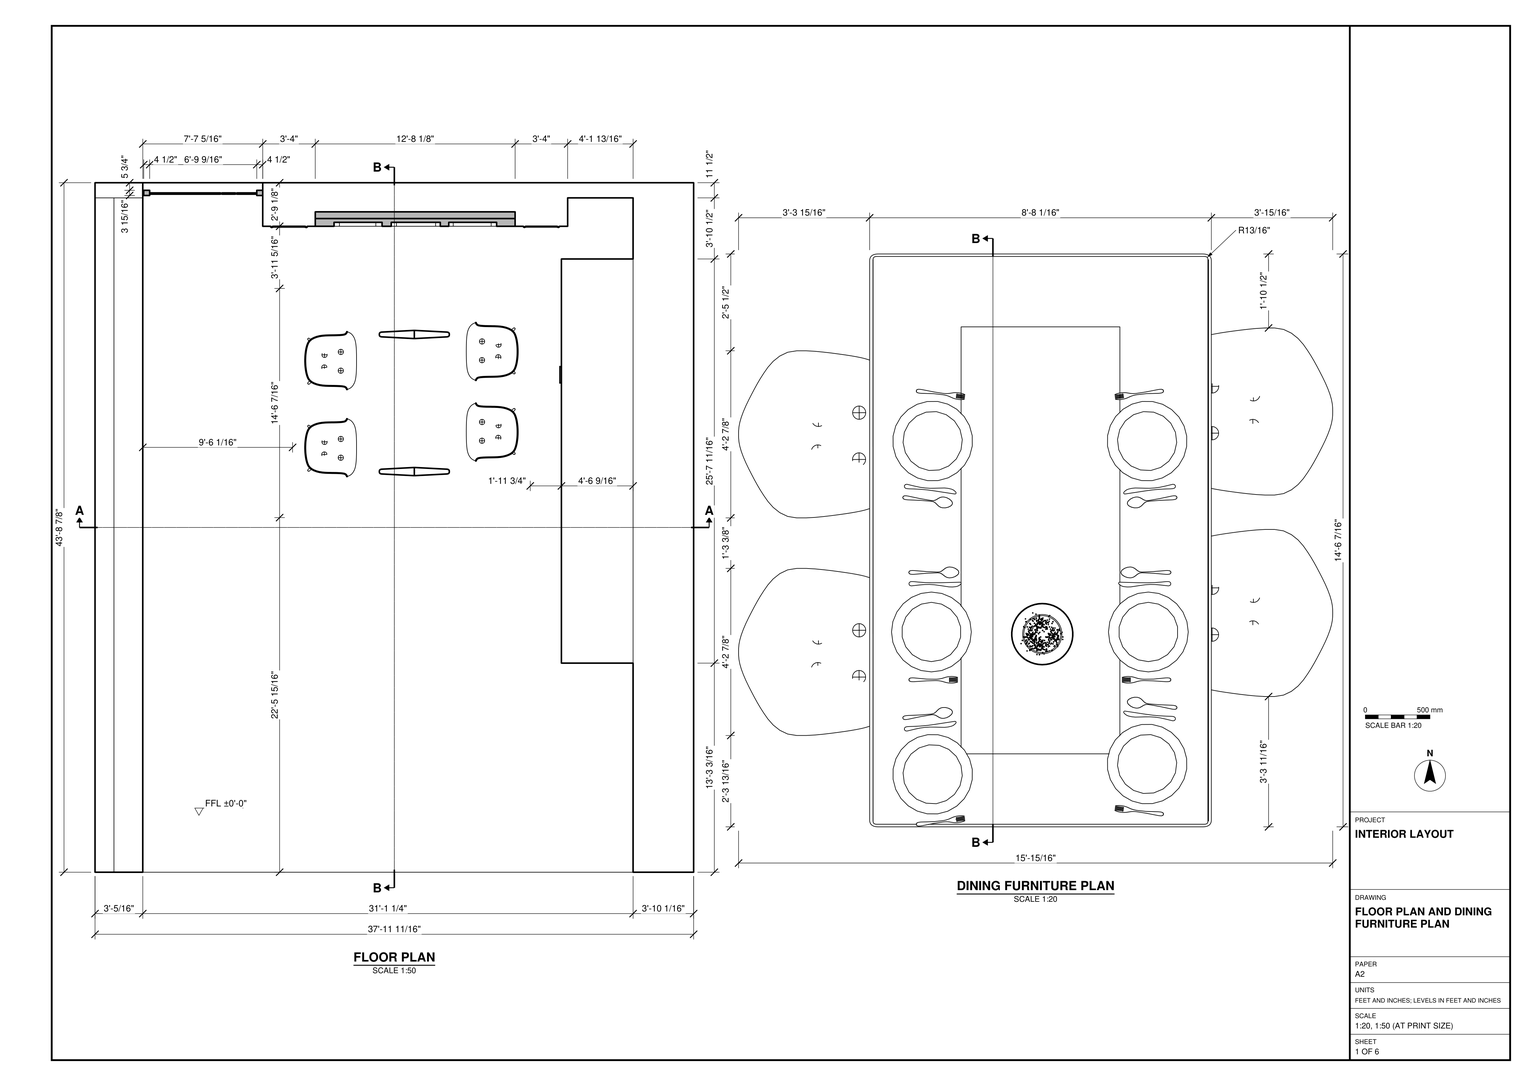
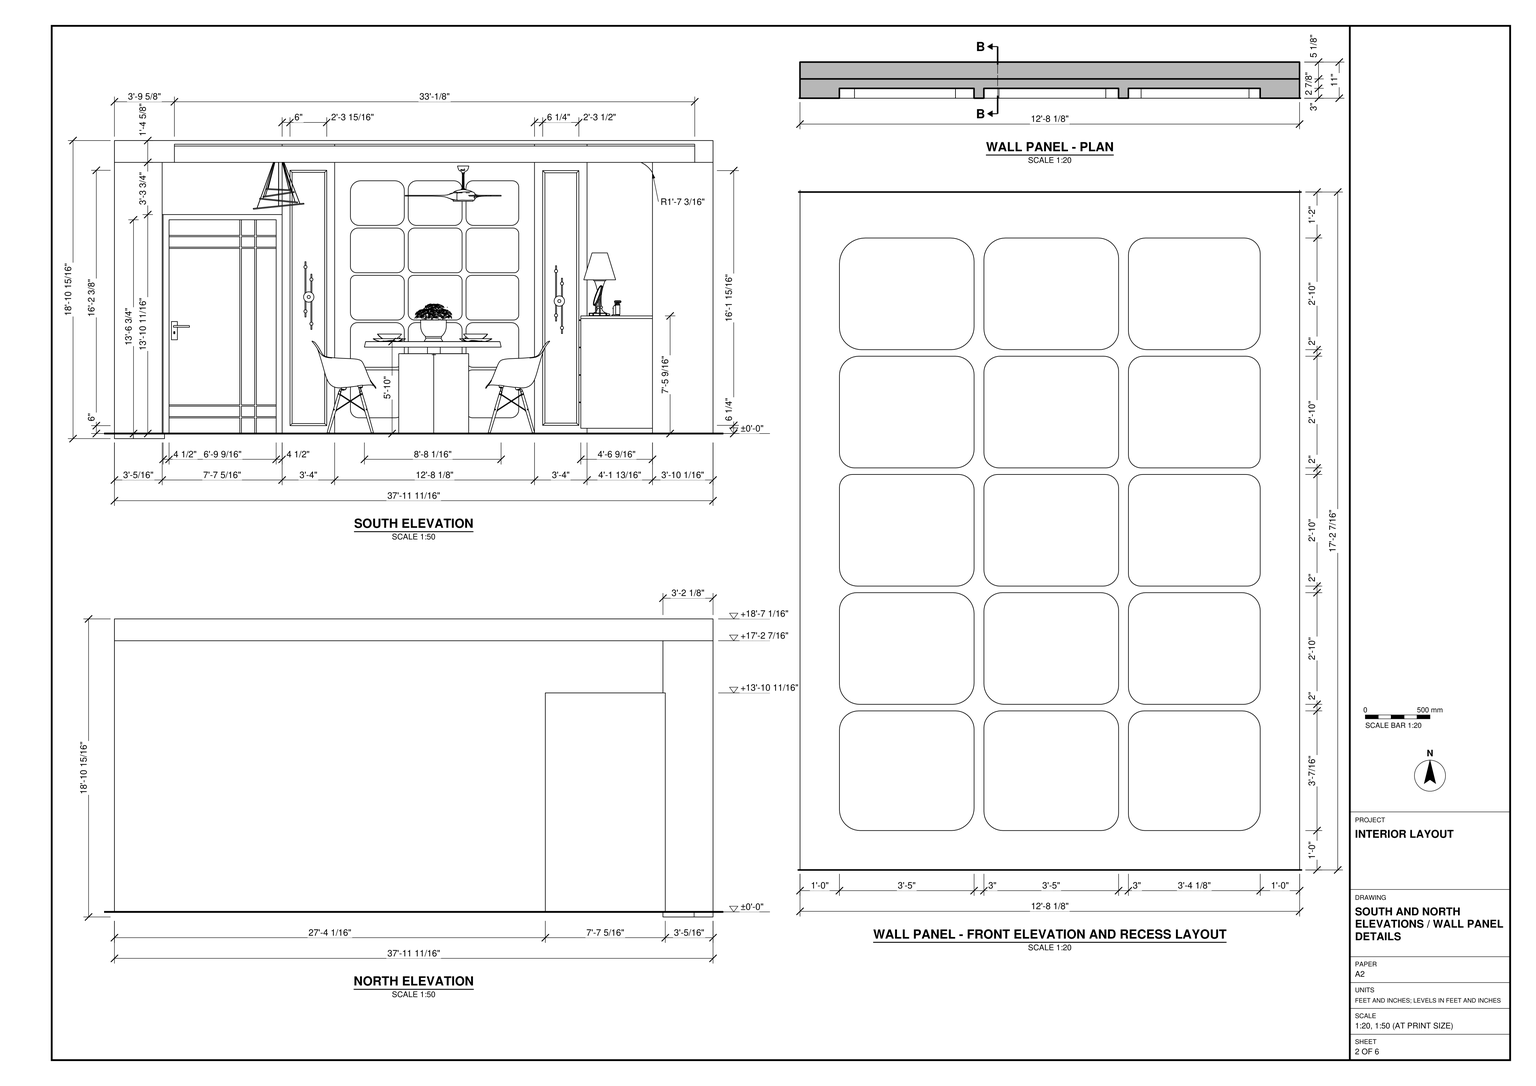
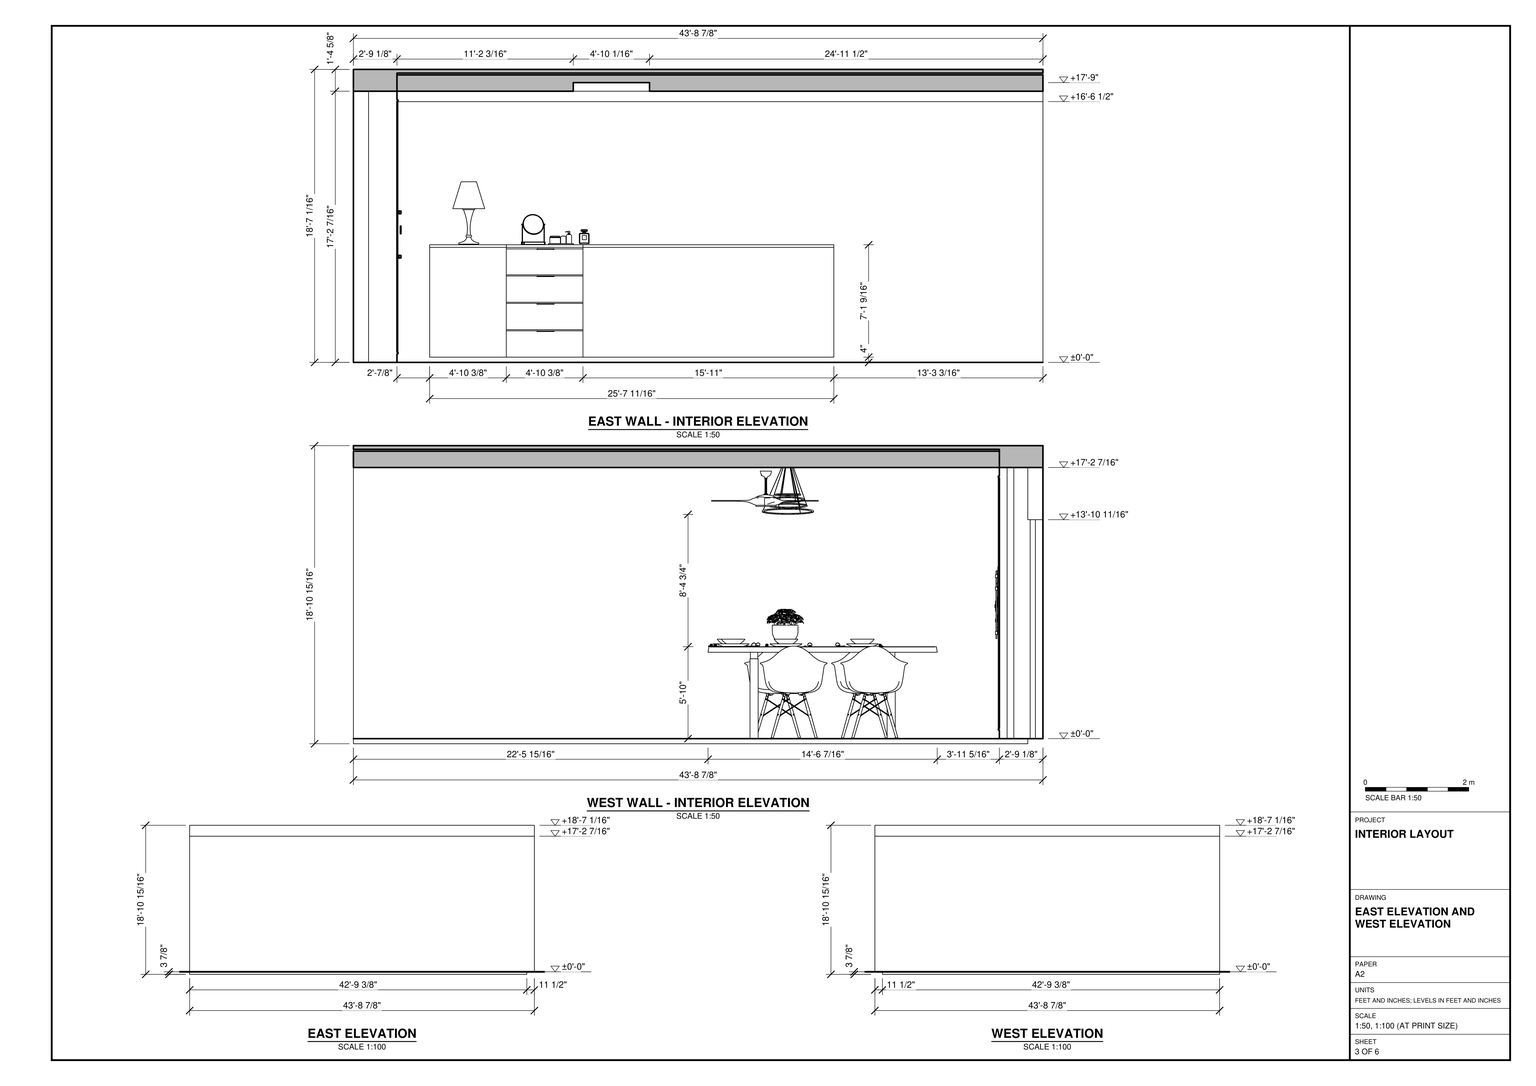
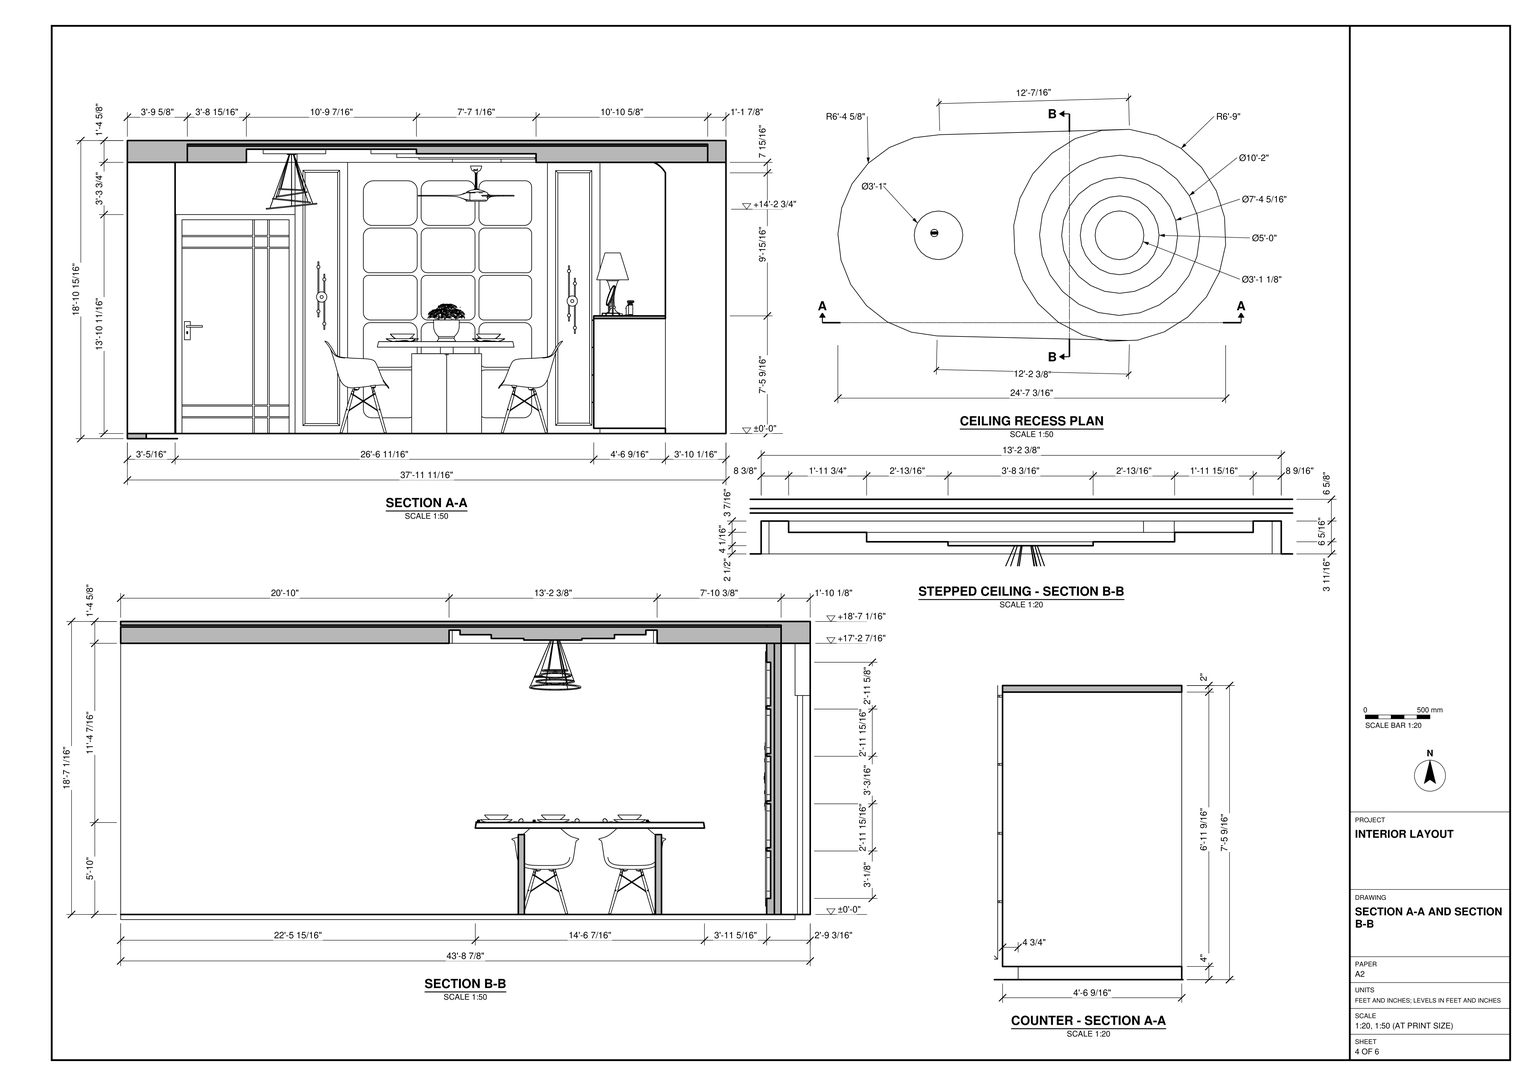
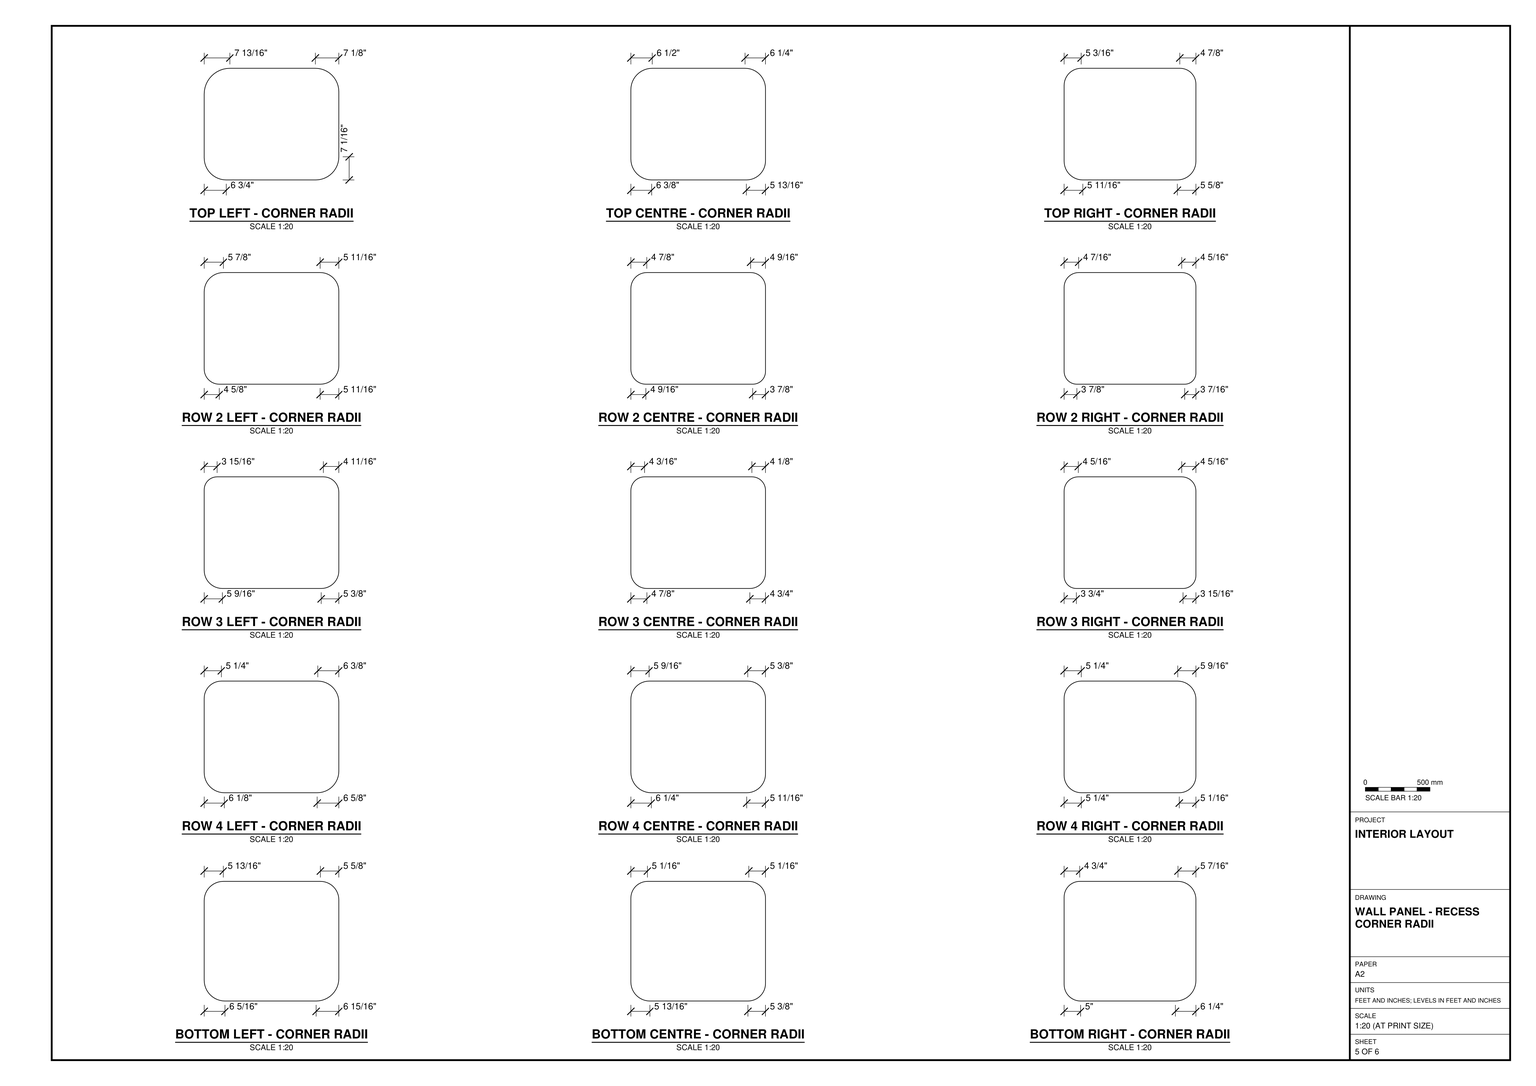
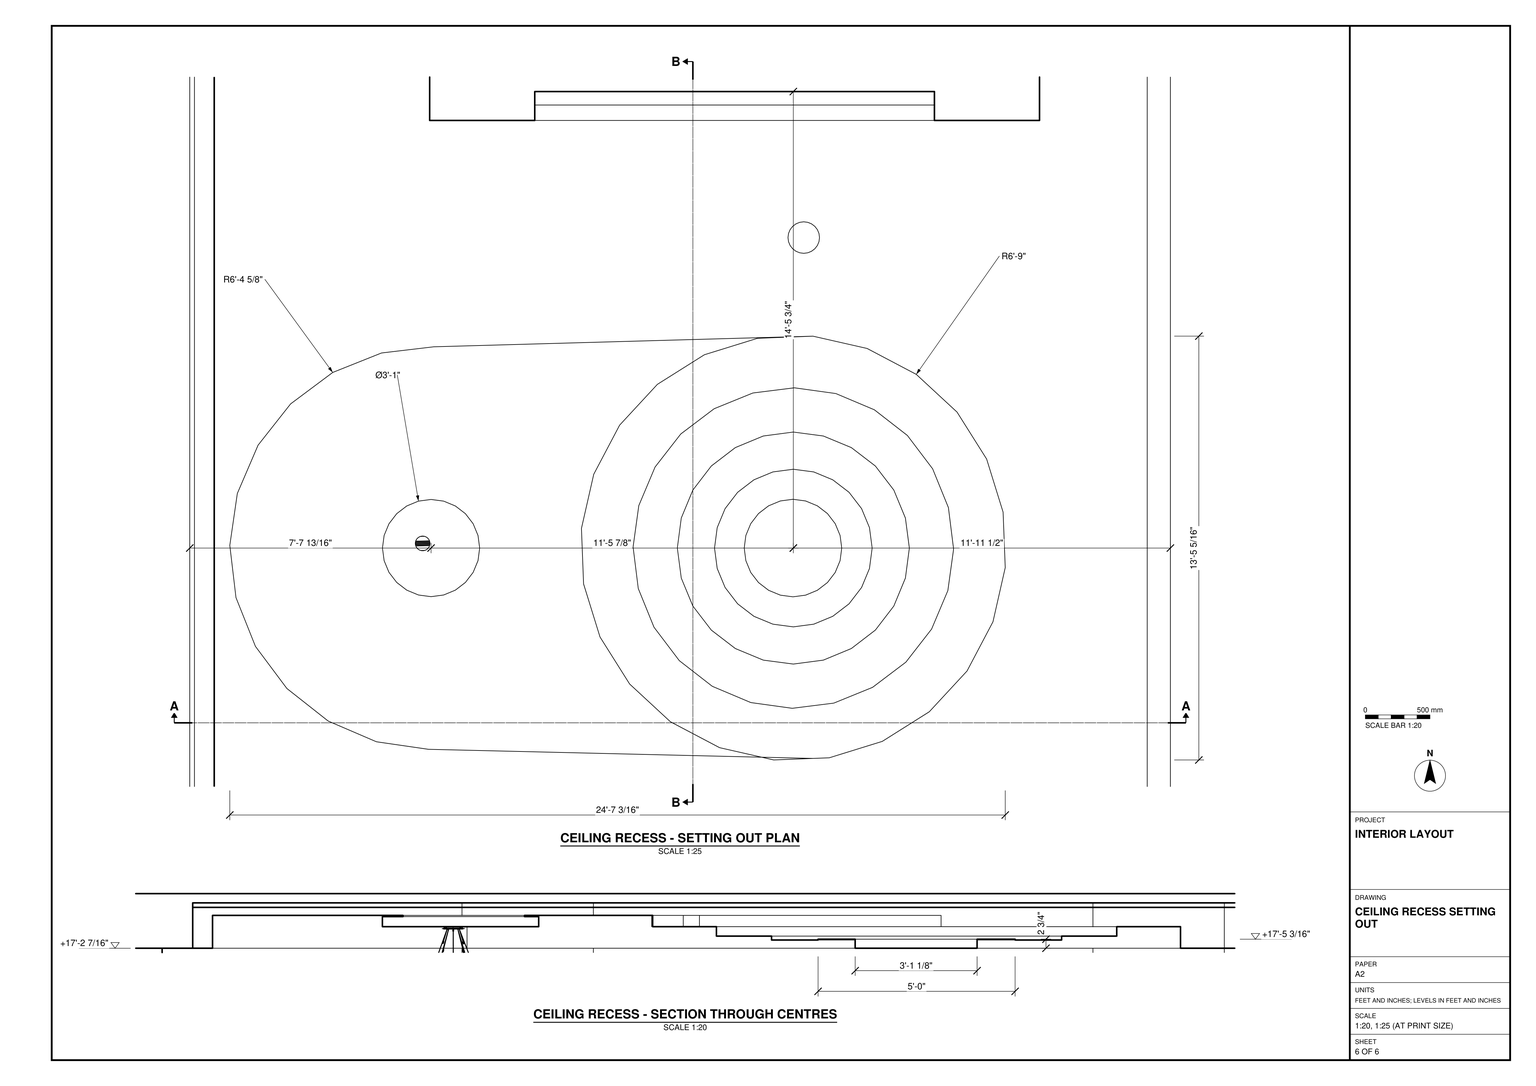
Build the dining room in SketchUp from task_files/diagram_01.pdf. Work in feet and inches. The overall model is 37'-11 11/16" wide, 43'-8 7/8" deep and 18'-10 15/16" high, with a single finished floor level at ±0'-0".

Use the floor plan to set out the walls at their drawn thicknesses, and use the elevations to form the floor, overhead slab and changes in wall depth. At the dining end, model the door and its frame beside the feature wall. Give the central wall panel its grid of rounded rectangular recesses and the narrow framed panels on either side. Along the east wall, build the long cabinet with its continuous top, drawer stack and plain front sections.

Position the rectangular dining table with its short end facing the feature wall, leaving the larger area of clear floor at the opposite end of the room. Use the enlarged furniture plan for the chairs and place settings, and the elevations for the table height and overhead fixtures. Decor and loose items, including lamps, the ceiling fan, tableware and plants, may be any suitable library components.

Keep shell elements and individual furniture and joinery pieces in separate groups or components, and use components for repeated parts. Save one SketchUp model as output_files/dining_room_with_a_recessed_feature_wall.skp.

# SketchUp Ruby script. Lengths in inches.
U = 1.inch
M = Sketchup.active_model
def pt(a) = Geom::Point3d.new(a.map { |v| v * U })
def face(e, loops, mat)
  f = e.add_face(loops[0].map { |a| pt(a) })
  loops[1..].each { |l| e.add_face(l.map { |a| pt(a) }).erase! }
  f.material = f.back_material = mat if mat
  f
end
# faces: each face lists its corners as indices into pts; further lists are holes
def faces(e, pts, list, mat = nil) = list.each { |f| face(e, (f[0].is_a?(Array) ? f : [f]).map { |l| l.map { |i| pts[i] } }, mat) }
# xy, xz, yz: faces in a plane at the given z, y or x. An outline is a flat list of corners, or four numbers for a rectangle; further outlines are holes
def ring(l) = l.size == 4 ? [[l[0], l[1]], [l[2], l[1]], [l[2], l[3]], [l[0], l[3]]] : l.each_slice(2).to_a
def flat(e, list, mat, &to3) = list.each { |f| face(e, (f[0].is_a?(Array) ? f : [f]).map { |l| ring(l).map { |u, v| to3.(u, v) } }, mat) }
def xy(e, z, list, mat = nil) = flat(e, list, mat) { |x, y| [x, y, z] }
def xz(e, y, list, mat = nil) = flat(e, list, mat) { |x, z| [x, y, z] }
def yz(e, x, list, mat = nil) = flat(e, list, mat) { |y, z| [x, y, z] }
def lines(e, pts, list) = list.each { |a, b| e.add_line(pt(pts[a]), pt(pts[b])) }
# prism: a flat outline (further loops are holes) pulled along v
def prism(e, loops, v, mat = nil)
  f = face(e, loops, mat); d = Geom::Vector3d.new(v.map { |x| x * U })
  f.pushpull(f.normal.samedirection?(d) ? d.length : -d.length)
end
def box(e, o, s, mat = nil) = prism(e, [[o, [o[0] + s[0], o[1], o[2]], [o[0] + s[0], o[1] + s[1], o[2]], [o[0], o[1] + s[1], o[2]]]], [0, 0, s[2]], mat)
def at(x, y, z, deg = 0) = Geom::Transformation.translation(pt([x, y, z])) * Geom::Transformation.rotation(ORIGIN, Z_AXIS, deg.degrees)
def axes(o, x, y, z) = Geom::Transformation.new([*x, 0, *y, 0, *z, 0, *pt(o).to_a, 1])
def part(name) = M.definitions.add(name)
# library, detail: a bought-in or finely detailed component or shape, given as its bounding box
def library(name, o, s) = part(name).tap { |d| box(d.entities, o, s) }
def detail(e, o, s) = box(e.add_group.entities, o, s)
def put(e, d, t, mat = nil) = e.add_instance(d, t).tap { |i| i.material = mat if mat }
def group(e, t, mat = nil) = e.add_group.tap { |g| g.transformation = t; g.material = mat if mat }.entities
root = M.entities
M.materials.add("[0116_Lavender]").color = [230, 230, 250]
M.materials.add("[Color J01]2").color = [122, 110, 137]
M.materials.add("[Color M01]").color = [226, 226, 226]
M.materials.add("[Color M02]").color = [198, 198, 198]
M.materials.add("[Color M07]").color = [58, 58, 58]
M.materials.add("[Color M08]").color = [30, 30, 30]
M.materials.add("[Metal Corrugated Shiny]").color = [53, 53, 53]
c1 = part("Group\#46")
prism(c1.entities,[[[0.55,0,1.11],[0.51,0,1.03],[0.44,0,0.97],[0.36,0,0.9375],[0.28,0,0.92],[0.19,0,0.9375],[0.11,0,0.97],[0.05,0,1.03],[0,0,1.11],[0,0,0],[0.55,0,0]]],[0,0.79,0])
c2 = part("Cabinet pull")
put(c2.entities,c1,axes([0,1.42,1.36],[0,0,-1],[1,0,0],[0,-1,0]),"[Color M08]")
g1 = group(c2.entities,at(0,1.42,1.36),"[Color M08]")
prism(g1,[[[0,-1.28,-0.57],[0,-1.32,-0.53],[0,-1.35,-0.49],[0,-1.38,-0.4375],[0,-1.4,-0.39],[0,-1.41,-0.33],[0,-1.42,-0.28],[0,-1.41,-0.22],[0,-1.4,-0.17],[0,-1.38,-0.11],[0,-1.35,-0.0625],[0,-1.32,-0.02],[0,-1.28,0.02],[0,-1.19,0.02],[0,-1.11,0],[0,-1.03,-0.05],[0,-0.97,-0.11],[0,-0.9375,-0.19],[0,-0.92,-0.28],[0,-0.9375,-0.36],[0,-0.97,-0.44],[0,-1.03,-0.51],[0,-1.11,-0.55],[0,-1.19,-0.57]]],[13.07,0,0])
put(c2.entities,c1,axes([12.28,1.42,1.36],[0,0,-1],[1,0,0],[0,-1,0]),"[Color M08]")
c3 = library("Untitled (23)",[0,0,0],[36,4.39,84])
c4 = library("Bathroom accessory set",[0,0,0],[18.8125,6.58,10.0625])
c5 = library("Tabletop vanity mirror",[-0.04,0,0],[13.32,7.875,17.05])
c6 = library("Perfume bottle",[0,0,0],[5.52,3.68,7.92])
c7 = library("lamp",[0,0,0],[9.82,9.84,19.44])
c8 = library("031_FANZART_Zen",[-27.59,-27.12,5.07],[46.53,51.77,17.09])
c9 = library("Group\#1",[0,0,0],[152.125,5.875,206.4375])
c10 = library("Group\#3",[0,0,0],[396.125,513.375,48.12])
c11 = part("Component\#2")
xy(c11.entities,0,[[3.9375,0,3.69,0.01,3.44,0.03,3.2,0.07,2.96,0.125,2.72,0.19,2.49,0.28,2.26,0.375,2.04,0.49,1.83,0.61,1.62,0.75,1.43,0.9,1.24,1.07,1.07,1.24,0.9,1.43,0.75,1.62,0.61,1.83,0.49,2.04,0.375,2.26,0.28,2.49,0.19,2.72,0.125,2.96,0.07,3.2,0.03,3.44,0.01,3.69,0,3.9375,0.01,4.18,0.03,4.43,0.07,4.67,0.125,4.92,0.19,5.15,0.28,5.39,0.375,5.61,0.49,5.83,0.61,6.05,0.75,6.25,0.9,6.45,1.24,6.81,1.43,6.97,1.62,7.12,1.83,7.26,2.04,7.39,2.26,7.5,2.49,7.6,2.72,7.68,2.96,7.75,3.2,7.8,3.44,7.84,3.69,7.87,3.9375,7.875,4.18,7.87,4.43,7.84,4.67,7.8,4.92,7.75,5.15,7.68,5.39,7.6,5.61,7.5,5.83,7.39,6.05,7.26,6.25,7.12,6.45,6.97,6.63,6.81,6.81,6.63,6.97,6.45,7.12,6.25,7.26,6.05,7.39,5.83,7.5,5.61,7.6,5.39,7.68,5.15,7.75,4.92,7.8,4.67,7.84,4.43,7.87,4.18,7.875,3.9375,7.87,3.69,7.84,3.44,7.8,3.2,7.75,2.96,7.68,2.72,7.6,2.49,7.5,2.26,7.39,2.04,7.26,1.83,7.12,1.62,6.97,1.43,6.81,1.24,6.45,0.9,6.25,0.75,6.05,0.61,5.83,0.49,5.61,0.375,5.39,0.28,5.15,0.19,4.92,0.125,4.67,0.07,4.43,0.03,4.18,0.01]])
xy(c11.entities,0.39,[[[3.9375,0,4.18,0.01,4.43,0.03,4.67,0.07,4.92,0.125,5.15,0.19,5.39,0.28,5.61,0.375,5.83,0.49,6.05,0.61,6.25,0.75,6.45,0.9,6.81,1.24,6.97,1.43,7.12,1.62,7.26,1.83,7.39,2.04,7.5,2.26,7.6,2.49,7.68,2.72,7.75,2.96,7.8,3.2,7.84,3.44,7.87,3.69,7.875,3.9375,7.87,4.18,7.84,4.43,7.8,4.67,7.75,4.92,7.68,5.15,7.6,5.39,7.5,5.61,7.39,5.83,7.26,6.05,7.12,6.25,6.97,6.45,6.81,6.63,6.63,6.81,6.45,6.97,6.25,7.12,6.05,7.26,5.83,7.39,5.61,7.5,5.39,7.6,5.15,7.68,4.92,7.75,4.67,7.8,4.43,7.84,4.18,7.87,3.9375,7.875,3.69,7.87,3.44,7.84,3.2,7.8,2.96,7.75,2.72,7.68,2.49,7.6,2.26,7.5,2.04,7.39,1.83,7.26,1.62,7.12,1.43,6.97,1.24,6.81,0.9,6.45,0.75,6.25,0.61,6.05,0.49,5.83,0.375,5.61,0.28,5.39,0.19,5.15,0.125,4.92,0.07,4.67,0.03,4.43,0.01,4.18,0,3.9375,0.01,3.69,0.03,3.44,0.07,3.2,0.125,2.96,0.19,2.72,0.28,2.49,0.375,2.26,0.49,2.04,0.61,1.83,0.75,1.62,0.9,1.43,1.07,1.24,1.24,1.07,1.43,0.9,1.62,0.75,1.83,0.61,2.04,0.49,2.26,0.375,2.49,0.28,2.72,0.19,2.96,0.125,3.2,0.07,3.44,0.03,3.69,0.01],[3.86,2.76,3.72,2.78,3.64,2.79,3.57,2.8125,3.5,2.84,3.43,2.87,3.37,2.9,3.3,2.94,3.24,2.98,3.18,3.03,3.03,3.18,2.98,3.24,2.94,3.3,2.9,3.37,2.87,3.43,2.84,3.5,2.8125,3.57,2.79,3.64,2.78,3.72,2.76,3.86,2.76,4.01,2.77,4.09,2.79,4.23,2.8125,4.3,2.84,4.37,2.9,4.51,2.98,4.63,3.08,4.75,3.18,4.85,3.3,4.93,3.37,4.97,3.43,5.01,3.5,5.04,3.64,5.08,3.72,5.1,3.86,5.12,4.01,5.12,4.09,5.11,4.16,5.1,4.37,5.04,4.44,5.01,4.51,4.97,4.69,4.85,4.75,4.8,4.8,4.75,4.85,4.69,4.97,4.51,5.01,4.44,5.04,4.37,5.1,4.16,5.11,4.09,5.12,4.01,5.12,3.86,5.1,3.72,5.08,3.64,5.04,3.5,5.01,3.43,4.97,3.37,4.93,3.3,4.85,3.18,4.75,3.08,4.63,2.98,4.51,2.9,4.37,2.84,4.3,2.8125,4.23,2.79,4.09,2.77,4.01,2.76]],[3.86,2.76,4.01,2.76,4.09,2.77,4.23,2.79,4.3,2.8125,4.37,2.84,4.51,2.9,4.63,2.98,4.75,3.08,4.85,3.18,4.93,3.3,4.97,3.37,5.01,3.43,5.04,3.5,5.08,3.64,5.1,3.72,5.12,3.86,5.12,4.01,5.11,4.09,5.1,4.16,5.04,4.37,5.01,4.44,4.97,4.51,4.85,4.69,4.8,4.75,4.75,4.8,4.69,4.85,4.51,4.97,4.44,5.01,4.37,5.04,4.16,5.1,4.09,5.11,4.01,5.12,3.86,5.12,3.72,5.1,3.64,5.08,3.5,5.04,3.43,5.01,3.37,4.97,3.3,4.93,3.18,4.85,3.08,4.75,2.98,4.63,2.9,4.51,2.84,4.37,2.8125,4.3,2.79,4.23,2.77,4.09,2.76,4.01,2.76,3.86,2.78,3.72,2.79,3.64,2.8125,3.57,2.84,3.5,2.87,3.43,2.9,3.37,2.94,3.3,2.98,3.24,3.03,3.18,3.18,3.03,3.24,2.98,3.3,2.94,3.37,2.9,3.43,2.87,3.5,2.84,3.57,2.8125,3.64,2.79,3.72,2.78]])
p = [[3.2,0.07,0],[3.44,0.03,0],[3.44,0.03,0.39],[3.2,0.07,0.39],[3.69,0.01,0],[3.69,0.01,0.39],
  [3.9375,0,0],[3.9375,0,0.39],[4.18,0.01,0],[4.18,0.01,0.39],[4.43,0.03,0],[4.43,0.03,0.39],
  [4.67,0.07,0],[4.67,0.07,0.39],[2.72,0.19,0],[2.96,0.125,0],[2.96,0.125,0.39],[2.72,0.19,0.39],
  [4.92,0.125,0],[4.92,0.125,0.39],[5.15,0.19,0],[5.15,0.19,0.39],[2.49,0.28,0],[2.49,0.28,0.39],
  [5.39,0.28,0],[5.39,0.28,0.39],[2.26,0.375,0],[2.26,0.375,0.39],[5.61,0.375,0],[5.61,0.375,0.39],
  [2.04,0.49,0],[2.04,0.49,0.39],[5.83,0.49,0],[5.83,0.49,0.39],[1.83,0.61,0],[1.83,0.61,0.39],
  [6.05,0.61,0],[6.05,0.61,0.39],[1.62,0.75,0],[1.62,0.75,0.39],[6.25,0.75,0],[6.25,0.75,0.39],
  [1.43,0.9,0],[1.43,0.9,0.39],[6.45,0.9,0],[6.45,0.9,0.39],[1.24,1.07,0],[1.24,1.07,0.39],
  [6.63,1.07,0],[6.63,1.07,0.39],[1.07,1.24,0],[1.07,1.24,0.39],[6.81,1.24,0],[6.81,1.24,0.39],
  [0.9,1.43,0],[0.9,1.43,0.39],[6.97,1.43,0],[6.97,1.43,0.39],[0.75,1.62,0],[0.75,1.62,0.39],
  [7.12,1.62,0],[7.12,1.62,0.39],[0.61,1.83,0],[0.61,1.83,0.39],[7.26,1.83,0],[7.26,1.83,0.39],
  [0.49,2.04,0],[0.49,2.04,0.39],[7.39,2.04,0],[7.39,2.04,0.39],[0.375,2.26,0],[0.375,2.26,0.39],
  [7.5,2.26,0],[7.5,2.26,0.39],[0.28,2.49,0],[0.28,2.49,0.39],[7.6,2.49,0],[7.6,2.49,0.39],
  [0.19,2.72,0],[0.19,2.72,0.39],[7.68,2.72,0],[7.68,2.72,0.39],[0.125,2.96,0],[0.125,2.96,0.39],
  [7.75,2.96,0],[7.75,2.96,0.39],[0.07,3.2,0],[0.07,3.2,0.39],[7.8,3.2,0],[7.8,3.2,0.39],
  [0.03,3.44,0],[0.03,3.44,0.39],[7.84,3.44,0],[7.84,3.44,0.39],[0.01,3.69,0],[0.01,3.69,0.39],
  [7.87,3.69,0],[7.87,3.69,0.39],[0,3.9375,0],[0,3.9375,0.39],[7.875,3.9375,0],[7.875,3.9375,0.39],
  [0.01,4.18,0],[0.01,4.18,0.39],[7.87,4.18,0],[7.87,4.18,0.39],[0.03,4.43,0],[0.03,4.43,0.39],
  [7.84,4.43,0],[7.84,4.43,0.39],[0.07,4.67,0],[0.07,4.67,0.39],[7.8,4.67,0],[7.8,4.67,0.39],
  [0.125,4.92,0],[0.125,4.92,0.39],[7.75,4.92,0],[7.75,4.92,0.39],[0.19,5.15,0],[0.19,5.15,0.39],
  [7.68,5.15,0],[7.68,5.15,0.39],[0.28,5.39,0],[0.28,5.39,0.39],[7.6,5.39,0],[7.6,5.39,0.39],
  [0.375,5.61,0],[0.375,5.61,0.39],[7.5,5.61,0],[7.5,5.61,0.39],[0.49,5.83,0],[0.49,5.83,0.39],
  [7.39,5.83,0],[7.39,5.83,0.39],[0.61,6.05,0],[0.61,6.05,0.39],[7.26,6.05,0],[7.26,6.05,0.39],
  [0.75,6.25,0],[0.75,6.25,0.39],[7.12,6.25,0],[7.12,6.25,0.39],[0.9,6.45,0],[0.9,6.45,0.39],
  [6.97,6.45,0],[6.97,6.45,0.39],[1.07,6.63,0],[1.07,6.63,0.39],[6.81,6.63,0],[6.81,6.63,0.39],
  [1.24,6.81,0],[1.24,6.81,0.39],[6.63,6.81,0],[6.63,6.81,0.39],[1.43,6.97,0],[1.43,6.97,0.39],
  [6.45,6.97,0],[6.45,6.97,0.39],[1.62,7.12,0],[1.62,7.12,0.39],[6.25,7.12,0],[6.25,7.12,0.39],
  [1.83,7.26,0],[1.83,7.26,0.39],[6.05,7.26,0],[6.05,7.26,0.39],[2.04,7.39,0],[2.04,7.39,0.39],
  [5.83,7.39,0],[5.83,7.39,0.39],[2.26,7.5,0],[2.26,7.5,0.39],[5.61,7.5,0],[5.61,7.5,0.39],
  [2.49,7.6,0],[2.49,7.6,0.39],[5.39,7.6,0],[5.39,7.6,0.39],[2.72,7.68,0],[2.72,7.68,0.39],
  [5.15,7.68,0],[5.15,7.68,0.39],[2.96,7.75,0],[2.96,7.75,0.39],[4.92,7.75,0],[4.92,7.75,0.39],
  [3.2,7.8,0],[3.2,7.8,0.39],[3.44,7.84,0],[3.44,7.84,0.39],[3.69,7.87,0],[3.69,7.87,0.39],
  [4.43,7.84,0],[4.18,7.87,0],[4.18,7.87,0.39],[4.43,7.84,0.39],[4.67,7.8,0],[4.67,7.8,0.39],
  [3.9375,7.875,0],[3.9375,7.875,0.39]]
faces(c11.entities,p,[[0,1,2,3],[1,4,5,2],[4,6,7,5],[6,8,9,7],[8,10,11,9],[10,12,13,11],[14,15,16,17],[15,0,3,16],
  [12,18,19,13],[18,20,21,19],[22,14,17,23],[20,24,25,21],[26,22,23,27],[24,28,29,25],[30,26,27,31],[28,32,33,29],
  [34,30,31,35],[32,36,37,33],[38,34,35,39],[36,40,41,37],[42,38,39,43],[40,44,45,41],[46,42,43,47],[44,48,49,45],
  [50,46,47,51],[48,52,53,49],[54,50,51,55],[52,56,57,53],[58,54,55,59],[56,60,61,57],[62,58,59,63],[60,64,65,61],
  [66,62,63,67],[64,68,69,65],[70,66,67,71],[68,72,73,69],[74,70,71,75],[72,76,77,73],[78,74,75,79],[76,80,81,77],
  [82,78,79,83],[80,84,85,81],[86,82,83,87],[84,88,89,85],[90,86,87,91],[88,92,93,89],[94,90,91,95],[92,96,97,93],
  [98,94,95,99],[96,100,101,97],[102,98,99,103],[100,104,105,101],[106,102,103,107],[104,108,109,105],[110,106,107,111],[108,112,113,109],
  [114,110,111,115],[112,116,117,113],[118,114,115,119],[116,120,121,117],[122,118,119,123],[120,124,125,121],[126,122,123,127],[124,128,129,125],
  [130,126,127,131],[128,132,133,129],[134,130,131,135],[132,136,137,133],[138,134,135,139],[136,140,141,137],[142,138,139,143],[140,144,145,141],
  [146,142,143,147],[144,148,149,145],[150,146,147,151],[148,152,153,149],[154,150,151,155],[152,156,157,153],[158,154,155,159],[156,160,161,157],
  [162,158,159,163],[160,164,165,161],[166,162,163,167],[164,168,169,165],[170,166,167,171],[168,172,173,169],[174,170,171,175],[172,176,177,173],
  [178,174,175,179],[176,180,181,177],[182,178,179,183],[180,184,185,181],[186,182,183,187],[188,186,187,189],[190,188,189,191],[192,193,194,195],
  [196,192,195,197],[184,196,197,185],[198,190,191,199],[193,198,199,194]])
c12 = part("Group\#327")
prism(c12.entities,[[[0.01,1.03,-0.79],[0,1.11,-0.79],[0,1.18,-0.79],[0,1.26,-0.79],[0.01,1.33,-0.79],[0.02,1.4,-0.79],[0.04,1.47,-0.79],[0.06,1.55,-0.79],[0.08,1.62,-0.79],[0.11,1.68,-0.79],[0.15,1.75,-0.79],[0.18,1.8125,-0.79],[0.23,1.875,-0.79],[0.27,1.93,-0.79],[0.32,1.99,-0.79],[0.37,2.04,-0.79],[0.43,2.09,-0.79],[0.49,2.14,-0.79],[0.55,2.18,-0.79],[0.61,2.22,-0.79],[0.68,2.25,-0.79],[0.75,2.28,-0.79],[0.82,2.3,-0.79],[0.89,2.33,-0.79],[0.96,2.34,-0.79],[1.03,2.35,-0.79],[1.11,2.36,-0.79],[1.18,2.36,-0.79],[1.26,2.36,-0.79],[1.33,2.35,-0.79],[1.4,2.34,-0.79],[1.47,2.33,-0.79],[1.55,2.3,-0.79],[1.62,2.28,-0.79],[1.68,2.25,-0.79],[1.75,2.22,-0.79],[1.8125,2.18,-0.79],[1.875,2.14,-0.79],[1.93,2.09,-0.79],[1.99,2.04,-0.79],[2.04,1.99,-0.79],[2.09,1.93,-0.79],[2.14,1.875,-0.79],[2.18,1.8125,-0.79],[2.22,1.75,-0.79],[2.25,1.68,-0.79],[2.28,1.62,-0.79],[2.3,1.55,-0.79],[2.33,1.47,-0.79],[2.34,1.4,-0.79],[2.35,1.33,-0.79],[2.36,1.26,-0.79],[2.36,1.18,-0.79],[2.36,1.11,-0.79],[2.35,1.03,-0.79],[2.34,0.96,-0.79],[2.33,0.89,-0.79],[2.3,0.82,-0.79],[2.28,0.75,-0.79],[2.25,0.68,-0.79],[2.22,0.61,-0.79],[2.18,0.55,-0.79],[2.14,0.49,-0.79],[2.09,0.43,-0.79],[2.04,0.37,-0.79],[1.99,0.32,-0.79],[1.93,0.27,-0.79],[1.875,0.23,-0.79],[1.8125,0.18,-0.79],[1.75,0.15,-0.79],[1.68,0.11,-0.79],[1.62,0.08,-0.79],[1.55,0.06,-0.79],[1.47,0.04,-0.79],[1.4,0.02,-0.79],[1.33,0.01,-0.79],[1.26,0,-0.79],[1.18,0,-0.79],[1.11,0,-0.79],[1.03,0.01,-0.79],[0.96,0.02,-0.79],[0.89,0.04,-0.79],[0.82,0.06,-0.79],[0.75,0.08,-0.79],[0.68,0.11,-0.79],[0.61,0.15,-0.79],[0.55,0.18,-0.79],[0.49,0.23,-0.79],[0.43,0.27,-0.79],[0.37,0.32,-0.79],[0.32,0.37,-0.79],[0.27,0.43,-0.79],[0.23,0.49,-0.79],[0.18,0.55,-0.79],[0.15,0.61,-0.79],[0.11,0.68,-0.79],[0.08,0.75,-0.79],[0.06,0.82,-0.79],[0.04,0.89,-0.79],[0.02,0.96,-0.79]]],[0,0,1.57],"[Metal Corrugated Shiny]")
c13 = part("Group\#324")
prism(c13.entities,[[[0.73,0.2,0],[0.67,0.12,0],[0.59,0.05,0],[0.5,0.01,0],[0.39,0,0],[0.29,0.01,0],[0.2,0.05,0],[0.12,0.12,0],[0.05,0.2,0],[0.01,0.29,0],[0,0.39,0],[0.01,0.5,0],[0.05,0.59,0],[0.12,0.67,0],[0.2,0.73,0],[0.29,0.77,0],[0.39,0.79,0],[0.5,0.77,0],[0.59,0.73,0],[0.67,0.67,0],[0.73,0.59,0],[0.77,0.5,0],[0.79,0.39,0],[0.77,0.29,0]]],[0,0,42.125],"[Metal Corrugated Shiny]")
c14 = part("Group\#4")
put(c14.entities,c11,axes([0,0.79,20.79],[1,0,0],[0,0,1],[0,-1,0]),"[Color M07]")
put(c14.entities,c12,axes([4.77,1.18,36.89],[1,0,0],[0,0,1],[0,-1,0]))
put(c14.entities,c12,axes([0.26,1.18,46.37],[1,0,0],[0,0,1],[0,-1,0]))
put(c14.entities,c12,axes([0.26,1.18,12.63],[1,0,0],[0,0,1],[0,-1,0]))
g2 = group(c14.entities,at(2.76,0.39,23.54))
prism(g2,[[[0.01,0,1.03],[0,0,1.11],[0,0,1.18],[0,0,1.26],[0.01,0,1.33],[0.02,0,1.4],[0.04,0,1.47],[0.06,0,1.55],[0.08,0,1.62],[0.11,0,1.68],[0.15,0,1.75],[0.18,0,1.8125],[0.23,0,1.875],[0.27,0,1.93],[0.32,0,1.99],[0.37,0,2.04],[0.43,0,2.09],[0.49,0,2.14],[0.55,0,2.18],[0.61,0,2.22],[0.68,0,2.25],[0.75,0,2.28],[0.82,0,2.3],[0.89,0,2.33],[0.96,0,2.34],[1.03,0,2.35],[1.11,0,2.36],[1.18,0,2.36],[1.26,0,2.36],[1.33,0,2.35],[1.4,0,2.34],[1.47,0,2.33],[1.55,0,2.3],[1.62,0,2.28],[1.68,0,2.25],[1.75,0,2.22],[1.8125,0,2.18],[1.875,0,2.14],[1.93,0,2.09],[1.99,0,2.04],[2.04,0,1.99],[2.09,0,1.93],[2.14,0,1.875],[2.18,0,1.8125],[2.22,0,1.75],[2.25,0,1.68],[2.28,0,1.62],[2.3,0,1.55],[2.33,0,1.47],[2.34,0,1.4],[2.35,0,1.33],[2.36,0,1.26],[2.36,0,1.18],[2.36,0,1.11],[2.35,0,1.03],[2.34,0,0.96],[2.33,0,0.89],[2.3,0,0.82],[2.28,0,0.75],[2.25,0,0.68],[2.22,0,0.61],[2.18,0,0.55],[2.14,0,0.49],[2.09,0,0.43],[2.04,0,0.37],[1.99,0,0.32],[1.93,0,0.27],[1.875,0,0.23],[1.8125,0,0.18],[1.75,0,0.15],[1.68,0,0.11],[1.62,0,0.08],[1.55,0,0.06],[1.47,0,0.04],[1.4,0,0.02],[1.33,0,0.01],[1.26,0,0],[1.18,0,0],[1.11,0,0],[1.03,0,0.01],[0.96,0,0.02],[0.89,0,0.04],[0.82,0,0.06],[0.75,0,0.08],[0.68,0,0.11],[0.61,0,0.15],[0.55,0,0.18],[0.49,0,0.23],[0.43,0,0.27],[0.37,0,0.32],[0.32,0,0.37],[0.27,0,0.43],[0.23,0,0.49],[0.18,0,0.55],[0.15,0,0.61],[0.11,0,0.68],[0.08,0,0.75],[0.06,0,0.82],[0.04,0,0.89],[0.02,0,0.96]]],[0,-0.39,0],"[Metal Corrugated Shiny]")
put(c14.entities,c13,at(1.05,0.79,9.48))
put(c14.entities,c12,axes([4.77,1.18,3.15],[1,0,0],[0,0,1],[0,-1,0]))
put(c14.entities,c13,at(5.56,0.79,0))
c15 = library("Group\#22",[0,-0.85,0],[159.52,154.66,89.09])
xy(root,-3.875,[[0,0,38.125,513.375]])
xy(root,0,[[0,0,14.41,513.375],[14.41,0,36.34,513.375],[36.34,0,409.59,0,409.59,513.375,359.78,513.375,359.78,491.75,319.78,491.75,319.78,502.75,167.66,502.75,167.66,491.75,127.66,491.75,127.66,524.91,36.34,524.91],[409.59,0,455.6875,0,455.6875,524.91,127.66,524.91,127.66,491.75,167.66,491.75,167.66,502.75,319.78,502.75,319.78,491.75,359.78,491.75,359.78,513.375,409.59,513.375],[0,513.375,36.34,524.91]])
xy(root,4,[[355.03,159.1875,409.59,466.85]])
xy(root,87.5625,[[355.03,159.1875,409.59,466.85]])
xy(root,89.5625,[[355.03,159.1875,409.59,466.85]])
xy(root,166.72,[[36.34,513.375,127.66,524.91]])
xy(root,200.41,[[133.68,491.52,161.63,491.52,161.625,491.75,133.6875,491.75]])
xy(root,206.4375,[[0,0,36.34,0,36.34,513.375,38.125,513.375,38.125,524.91,0,524.91],[36.34,0,38.125,513.375],[38.125,0,45.66,513.375],[441.78,0,441.78,513.375,359.78,513.375,359.78,491.75,319.78,491.75,319.78,502.75,167.66,502.75,167.66,491.75,127.66,491.75,127.66,513.375,38.125,513.375,38.125,524.91,455.6875,524.91,455.6875,0],[400.78,0,409.59,513.375],
  [409.59,0,441.78,513.375]])
xy(root,220.25,[[45.66,0,45.66,513.375,127.66,513.375,127.66,491.75,167.66,491.75,167.66,502.75,319.78,502.75,319.78,491.75,359.78,491.75,359.78,513.375,441.78,513.375,441.78,0]])
xy(root,223.0625,[[0,0,455.6875,524.91]])
xz(root,0,[[0,-3.875,14.41,0],[14.41,-3.875,38.125,0],[0,0,36.34,206.4375],[409.59,0,455.6875,206.4375],[409.59,198.52,409.59,206.4375,400.78,206.4375,401.6875,206.01,402.57,205.53,403.43,205.01,404.25,204.4375,405.05,203.83,405.8125,203.18,406.54,202.49,407.23,201.76,407.89,201,408.5,200.2,409.07,199.38],
  [0,206.4375,45.66,206.4375,45.66,220.25,441.78,220.25,441.78,206.4375,455.6875,206.4375,455.6875,223.0625,0,223.0625]])
xz(root,159.1875,[[355.03,4,409.59,87.5625],[355.03,87.5625,409.59,89.5625]])
xz(root,466.85,[[355.03,4,409.59,87.5625],[355.03,87.5625,409.59,89.5625]])
xz(root,491.75,[[127.66,206.4375,167.66,220.25],[319.78,206.4375,359.78,220.25]])
xz(root,491.75,[[[127.66,0,167.66,206.4375],[133.6875,6.03,161.625,200.41]],[[319.78,0,359.78,206.4375],[326.02,6.24,353.54,200.2]],[135.25,7.59,160.0625,198.84],[327.71,7.93,351.86,198.51]],"[Color M02]")
xz(root,502.75,[[167.66,0,319.78,206.4375],[167.66,206.4375,319.78,220.25]])
xz(root,513.375,[[0,-3.875,14.41,0],[45.66,206.4375,127.66,220.25],[359.78,206.4375,441.78,220.25]])
xz(root,513.375,[[359.78,0,409.59,0,409.59,198.52,409.07,199.38,408.5,200.2,407.89,201,407.23,201.76,406.54,202.49,405.8125,203.18,405.05,203.83,404.25,204.4375,403.43,205.01,402.57,205.53,401.6875,206.01,400.78,206.4375,359.78,206.4375],[36.34,166.72,127.66,206.4375]],"[Color J01]2")
xz(root,524.91,[[0,0,0,206.4375,38.125,206.4375,38.125,166.72,36.34,166.72,36.34,0],[36.34,0,127.66,166.72],[127.66,0,127.66,166.72,38.125,166.72,38.125,206.4375,455.6875,206.4375,455.6875,0],[0,206.4375,455.6875,223.0625]])
yz(root,0,[[0,-3.875,513.375,0],[0,0,524.91,206.4375],[0,206.4375,524.91,223.0625]])
yz(root,14.41,[[0,-3.875,513.375,0]])
yz(root,36.34,[[0,0,524.91,0,524.91,166.72,513.375,166.72,513.375,206.4375,0,206.4375]])
yz(root,45.66,[[0,206.4375,513.375,220.25]])
yz(root,127.66,[[491.75,0,491.75,206.4375,513.375,206.4375,513.375,166.72,524.91,166.72,524.91,0],[491.75,206.4375,513.375,220.25]])
yz(root,167.66,[[491.75,0,502.75,206.4375],[491.75,206.4375,502.75,220.25]])
yz(root,319.78,[[491.75,0,502.75,206.4375],[491.75,206.4375,502.75,220.25]])
yz(root,355.03,[[159.1875,4,350.16,87.5625],[408.5,4,466.85,87.5625],[159.1875,87.5625,350.16,89.5625],[350.16,87.5625,408.5,89.5625],[408.5,87.5625,466.85,89.5625]])
yz(root,355.03,[[350.16,4,408.5,24.02],[350.16,24.89,408.5,44.91],[350.16,45.78,408.5,65.8],[350.16,66.67,408.5,86.39]],"[Color J01]2")
yz(root,355.03,[[350.16,24.02,408.5,24.89],[350.16,44.91,408.5,45.78],[350.16,65.8,408.5,66.67],[350.16,86.39,408.5,87.5625]],"[Color M07]")
yz(root,359.78,[[491.75,0,513.375,206.4375],[491.75,206.4375,513.375,220.25]])
yz(root,409.59,[[159.1875,87.5625,466.85,89.5625]])
yz(root,409.59,[[[0,0,513.375,198.52],[159.1875,4,466.85,89.5625]]],"[Color J01]2")
yz(root,441.78,[[0,206.4375,513.375,220.25]])
yz(root,455.6875,[[0,0,524.91,206.4375],[0,206.4375,524.91,223.0625]])
p = [[133.68,491.52,6.02],[133.74,491.29,6.08],[133.74,491.29,200.35],[133.68,491.52,200.41],[161.63,491.52,6.02],[161.57,491.29,6.08],
  [161.63,491.52,200.41],[161.57,491.29,200.35],[133.6875,491.75,6.03],[133.6875,491.75,200.41],[161.625,491.75,6.03],[161.625,491.75,200.41],
  [133.86,491.1,6.2],[133.86,491.1,200.23],[161.45,491.1,6.2],[161.45,491.1,200.23],[134.03,490.94,6.375],[134.03,490.94,200.0625],
  [161.28,490.94,6.375],[161.28,490.94,200.0625],[326.02,491.75,6.24],[326.05,491.53,6.27],[326.05,491.53,200.17],[326.02,491.75,200.2],
  [353.54,491.75,6.24],[353.51,491.53,6.27],[327.71,491.53,6.27],[327.71,491.75,6.24],[353.54,491.75,200.2],[353.51,491.53,200.17],
  [326.13,491.33,6.35],[326.13,491.33,200.09],[327.71,491.33,6.35],[353.43,491.33,6.35],[353.43,491.33,200.09],[134.24,490.85,6.58],
  [134.24,490.85,199.85],[161.07,490.85,6.58],[161.07,490.85,199.85],[326.27,491.15,6.49],[326.27,491.15,199.95],[327.71,491.15,6.49],
  [353.3,491.15,6.49],[353.3,491.15,199.95],[326.44,491.02,6.66],[326.44,491.02,199.78],[353.12,491.02,6.66],[327.71,491.02,6.66],
  [353.12,491.02,199.78],[134.47,490.8125,6.8125],[134.47,490.8125,199.625],[160.84,490.8125,6.8125],[160.84,490.8125,199.625],[326.65,490.93,6.86],
  [326.65,490.93,199.57],[352.92,490.93,6.86],[327.71,490.93,6.86],[352.92,490.93,199.57],[134.7,490.85,7.04],[134.7,490.85,199.4],
  [160.61,490.85,7.04],[160.61,490.85,199.4],[326.86,490.91,7.08],[326.86,490.91,199.36],[352.7,490.91,7.08],[327.71,490.91,7.08],
  [352.7,490.91,199.36],[134.91,490.94,7.25],[134.91,490.94,199.1875],[160.4,490.94,7.25],[160.4,490.94,199.1875],[327.08,490.93,7.3],
  [327.08,490.93,199.14],[352.48,490.93,7.3],[327.71,490.93,7.3],[352.48,490.93,199.14],[135.08,491.1,7.42],[135.08,491.1,199.01],
  [160.23,491.1,7.42],[160.23,491.1,199.01],[327.29,491.02,7.5],[327.29,491.02,198.93],[352.28,491.02,7.5],[327.71,491.02,7.5],
  [352.28,491.02,198.93],[135.2,491.29,7.54],[135.2,491.29,198.89],[160.11,491.29,7.54],[160.11,491.29,198.89],[327.46,491.15,7.68],
  [327.46,491.15,198.76],[352.1,491.15,7.68],[327.71,491.15,7.68],[352.1,491.15,198.76],[135.26,491.52,7.6],[135.26,491.52,198.83],
  [160.05,491.52,7.6],[160.05,491.52,198.83],[135.25,491.75,7.59],[135.25,491.75,198.84],[160.0625,491.75,7.59],[160.0625,491.75,198.84],
  [327.59,491.33,7.8125],[327.59,491.33,198.625],[351.97,491.33,7.8125],[327.71,491.33,7.8125],[351.97,491.33,198.625],[327.68,491.53,7.9],
  [327.68,491.53,198.54],[327.71,491.53,7.9],[351.88,491.53,7.9],[351.88,491.53,198.54],[327.71,491.75,7.93],[327.71,491.75,198.51],
  [351.86,491.75,7.93],[351.86,491.75,198.51],[409.07,513.375,199.38],[409.59,513.375,198.52],[409.59,0,198.52],[409.07,0,199.38],
  [408.5,513.375,200.2],[408.5,0,200.2],[407.89,513.375,201],[407.89,0,201],[407.23,513.375,201.76],[407.23,0,201.76],
  [406.54,513.375,202.49],[406.54,0,202.49],[405.8125,513.375,203.18],[405.8125,0,203.18],[405.05,513.375,203.83],[405.05,0,203.83],
  [404.25,513.375,204.4375],[404.25,0,204.4375],[403.43,513.375,205.01],[403.43,0,205.01],[402.57,513.375,205.53],[402.57,0,205.53],
  [401.6875,513.375,206.01],[401.6875,0,206.01],[400.78,513.375,206.4375],[400.78,0,206.4375]]
faces(root,p,[[0,1,2,3],[4,5,1,0],[8,0,3,9],[10,4,0,8],[1,12,13,2],[5,14,12,1],[12,16,17,13],[14,18,16,12],
  [24,25,26,21,20,27],[32,30,21,26,25,33],[16,35,36,17],[18,37,35,16],[41,39,30,32,33,42],[42,46,47,44,39,41],[35,49,50,36],[37,51,49,35],
  [46,55,56,53,44,47],[49,58,59,50],[51,60,58,49],[55,64,65,62,53,56],[58,67,68,59],[60,69,67,58],[64,73,74,71,62,65],[67,76,77,68],
  [69,78,76,67],[73,82,83,80,71,74],[76,85,86,77],[78,87,85,76],[82,91,92,89,80,83],[85,94,95,86],[87,96,94,85],[94,98,99,95],
  [96,100,98,94],[91,104,105,102,89,92],[109,107,102,105,104,110],[112,107,109,110,114],[116,117,118,119],[103,108,111,106],[108,113,115,111],[90,103,106,93],
  [81,90,93,84],[86,95,97,88],[95,99,101,97],[72,81,84,75],[77,86,88,79],[68,77,79,70],[63,72,75,66],[59,68,70,61],
  [120,116,119,121],[50,59,61,52],[54,63,66,57],[36,50,52,38],[45,54,57,48],[40,45,48,43],[17,36,38,19],[31,40,43,34],
  [13,17,19,15],[22,31,34,29],[122,120,121,123],[2,13,15,7],[23,22,29,28],[3,2,7,6],[124,122,123,125],[126,124,125,127],
  [128,126,127,129],[130,128,129,131],[132,130,131,133],[134,132,133,135],[136,134,135,137],[138,136,137,139],[140,138,139,141]])
faces(root,p,[[6,7,5,4],[11,6,4,10],[7,15,14,5],[15,19,18,14],[19,38,37,18],[38,52,51,37],[52,61,60,51],[61,70,69,60],
  [70,79,78,69],[79,88,87,78],[88,97,96,87],[97,101,100,96]],"[Color M01]")
faces(root,p,[[20,21,22,23],[21,30,31,22],[30,39,40,31],[39,44,45,40],[44,53,54,45],[53,62,63,54],[62,71,72,63],[71,80,81,72],
  [80,89,90,81],[89,102,103,90],[102,107,108,103],[107,112,113,108]],"[Color M02]")
faces(root,p,[[28,29,25,24],[29,34,33,25],[34,43,42,33],[43,48,46,42],[48,57,55,46],[57,66,64,55],[66,75,73,64],[75,84,82,73],
  [84,93,91,82],[93,106,104,91],[106,111,110,104],[111,115,114,110]],"[0116_Lavender]")
put(root,c2,at(353.61,385.24,64.47,-90))
put(root,c2,at(353.61,385.24,43.47,-90))
put(root,c2,at(353.61,385.24,22.65,-90))
put(root,c2,at(353.61,385.24,85.22,-90))
put(root,c3,axes([37.06,514.75,0],[2.51667,0,0],[0,1,0],[0,0,1.9847]))
put(root,c4,axes([378.68,376.48,89.55],[0,-1.02,0],[1.02,0,0],[0,0,1.02]))
put(root,c5,axes([361.2,395.92,89.5625],[0.23616,-1.33934,0],[1.33934,0.23616,0],[0,0,1.36]))
put(root,c6,axes([380.63,352.95,90.35],[0,-1.36,0],[1.36,0,0],[0,0,1.36]))
put(root,c7,axes([357.3,424.95,89.5625],[2.4674,0,0],[0,2.4674,0],[0,0,2.4674]))
put(root,c8,axes([264.65,315.21,168.89],[1.57,0,0],[0,1.57,0],[0,0,1.57]))
put(root,c9,at(167.66,491.75,0),"[Color M02]")
put(root,c10,at(45.66,0,170.76),"[Color M01]")
put(root,c14,at(143.99,489.78,79.24))
put(root,c14,at(334.75,488.35,76.14))
put(root,c15,axes([150.38,269.97,0],[1.1342,0,0],[0,1.1342,0],[0,0,1.1342]))
